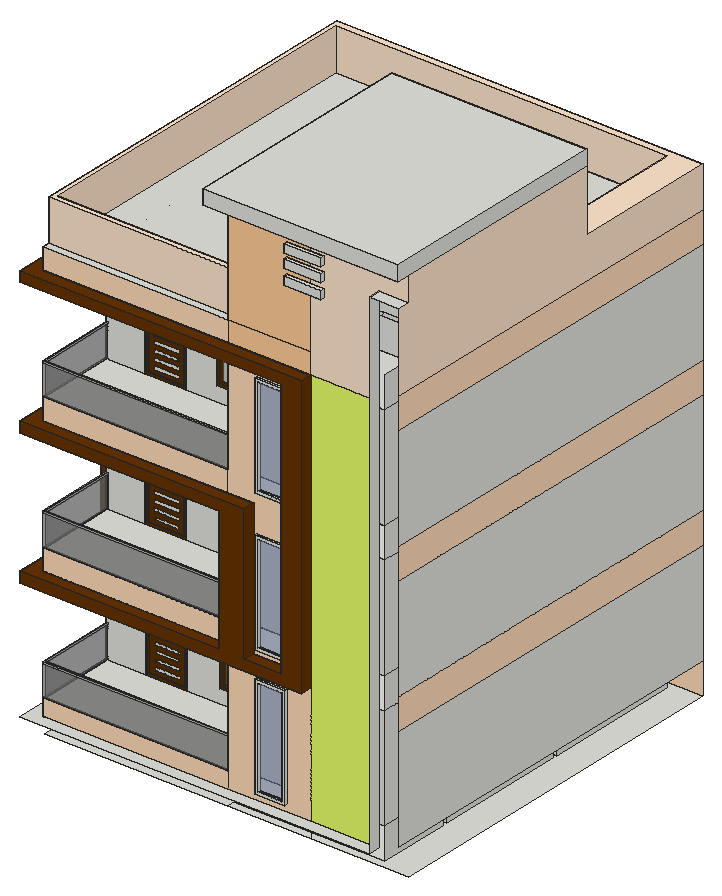
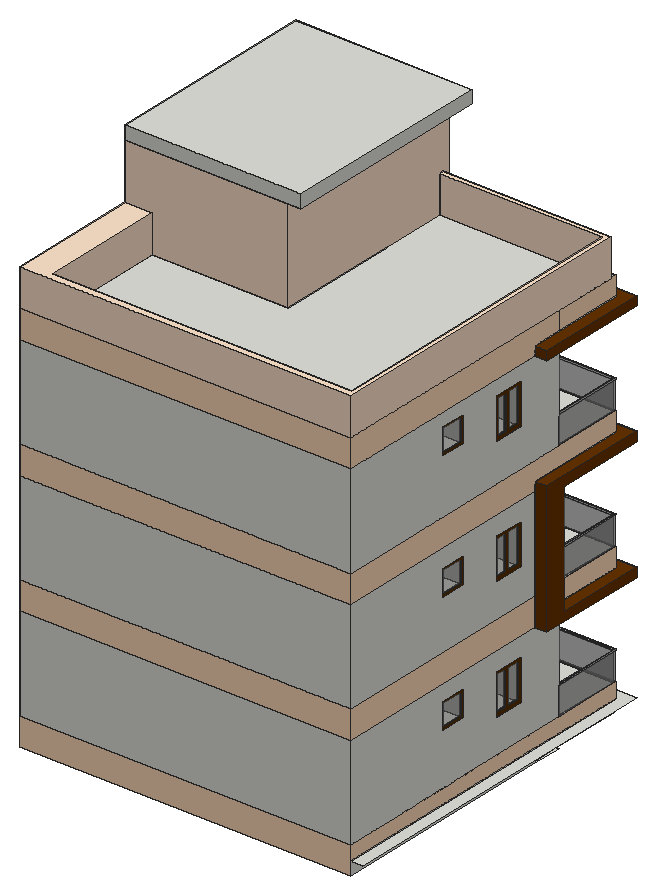
# SketchUp Ruby script. Lengths in inches.
U = 1.inch
M = Sketchup.active_model
def pt(a) = Geom::Point3d.new(a.map { |v| v * U })
def face(e, loops, mat)
  f = e.add_face(loops[0].map { |a| pt(a) })
  loops[1..].each { |l| e.add_face(l.map { |a| pt(a) }).erase! }
  f.material = f.back_material = mat if mat
  f
end
# faces: each face lists its corners as indices into pts; further lists are holes
def faces(e, pts, list, mat = nil) = list.each { |f| face(e, (f[0].is_a?(Array) ? f : [f]).map { |l| l.map { |i| pts[i] } }, mat) }
# xy, xz, yz: faces in a plane at the given z, y or x. An outline is a flat list of corners, or four numbers for a rectangle; further outlines are holes
def ring(l) = l.size == 4 ? [[l[0], l[1]], [l[2], l[1]], [l[2], l[3]], [l[0], l[3]]] : l.each_slice(2).to_a
def flat(e, list, mat, &to3) = list.each { |f| face(e, (f[0].is_a?(Array) ? f : [f]).map { |l| ring(l).map { |u, v| to3.(u, v) } }, mat) }
def xy(e, z, list, mat = nil) = flat(e, list, mat) { |x, y| [x, y, z] }
def xz(e, y, list, mat = nil) = flat(e, list, mat) { |x, z| [x, y, z] }
def yz(e, x, list, mat = nil) = flat(e, list, mat) { |y, z| [x, y, z] }
def lines(e, pts, list) = list.each { |a, b| e.add_line(pt(pts[a]), pt(pts[b])) }
# prism: a flat outline (further loops are holes) pulled along v
def prism(e, loops, v, mat = nil)
  f = face(e, loops, mat); d = Geom::Vector3d.new(v.map { |x| x * U })
  f.pushpull(f.normal.samedirection?(d) ? d.length : -d.length)
end
def box(e, o, s, mat = nil) = prism(e, [[o, [o[0] + s[0], o[1], o[2]], [o[0] + s[0], o[1] + s[1], o[2]], [o[0], o[1] + s[1], o[2]]]], [0, 0, s[2]], mat)
def at(x, y, z, deg = 0) = Geom::Transformation.translation(pt([x, y, z])) * Geom::Transformation.rotation(ORIGIN, Z_AXIS, deg.degrees)
def axes(o, x, y, z) = Geom::Transformation.new([*x, 0, *y, 0, *z, 0, *pt(o).to_a, 1])
def part(name) = M.definitions.add(name)
# library, detail: a bought-in or finely detailed component or shape, given as its bounding box
def library(name, o, s) = part(name).tap { |d| box(d.entities, o, s) }
def detail(e, o, s) = box(e.add_group.entities, o, s)
def put(e, d, t, mat = nil) = e.add_instance(d, t).tap { |i| i.material = mat if mat }
def group(e, t, mat = nil) = e.add_group.tap { |g| g.transformation = t; g.material = mat if mat }.entities
root = M.entities
M.materials.add("[0027_PeachPuff]").color = [255, 218, 185]
M.materials.add("[Aluminum]").color = [179, 179, 179]
M.materials.add("[Color A08]").color = [89, 48, 0]
M.materials.add("[Color C01]").color = [255, 229, 204]
M.materials.add("[Color C02]").color = [255, 204, 153]
M.materials.add("[Color C08]").color = [102, 51, 0]
M.materials.add("[Rectangles Running 4x1]").color = [231, 255, 106]
M.materials.add("[Translucent Glass Gray]").color = [128, 128, 128]
M.materials["[Translucent Glass Gray]"].alpha = 0.5
M.materials.add("[Translucent Glass Sky Reflection]").color = [126, 138, 183]
M.materials["[Translucent Glass Sky Reflection]"].alpha = 0.52
c1 = part("Group\#2")
xy(c1.entities,0,[[0,0,48,6.0625]],"[Color A08]")
xy(c1.entities,2.37,[[2.37,2.1875,45.63,6.0625]])
xy(c1.entities,2.37,[[2.37,0,45.63,2.1875]],"[Color A08]")
xy(c1.entities,81.63,[[2.37,2.1875,45.63,6.0625]])
xy(c1.entities,81.63,[[2.37,0,45.63,2.1875]],"[Color A08]")
xy(c1.entities,84,[[0,0,48,6.0625]],"[Color A08]")
xz(c1.entities,0,[[[0,0,48,84],[2.37,2.37,45.63,81.63]]],"[Color A08]")
xz(c1.entities,2.1875,[[9.64,6.54,37.83,9.91],[9.64,15.35,37.83,18.72],[9.64,24.16,37.83,27.54],[9.64,32.97,37.83,36.35],[9.64,41.79,37.83,45.16],
  [9.64,50.6,37.83,53.97],[9.64,59.41,37.83,62.79],[9.64,68.22,37.83,71.6]])
xz(c1.entities,2.1875,[[[2.37,2.37,45.63,81.63],[9.64,68.22,37.83,71.6],[9.64,59.41,37.83,62.79],[9.64,50.6,37.83,53.97],[9.64,41.79,37.83,45.16],[9.64,32.97,37.83,36.35],[9.64,24.16,37.83,27.54],[9.64,15.35,37.83,18.72],[9.64,6.54,37.83,9.91]]],"[Color A08]")
xz(c1.entities,6.0625,[[[0,0,48,84],[2.37,2.37,45.63,81.63]],[2.37,2.37,45.63,81.63]],"[Color A08]")
yz(c1.entities,0,[[0,0,6.0625,84]],"[Color A08]")
yz(c1.entities,2.37,[[2.1875,2.37,6.0625,81.63]])
yz(c1.entities,2.37,[[0,2.37,2.1875,81.63]],"[Color A08]")
yz(c1.entities,45.63,[[2.1875,2.37,6.0625,81.63]])
yz(c1.entities,45.63,[[0,2.37,2.1875,81.63]],"[Color A08]")
yz(c1.entities,48,[[0,0,6.0625,84]],"[Color A08]")
c2 = part("Group\#1")
xy(c2.entities,0,[[0,0,54.25,4.125]],"[Color A08]")
xy(c2.entities,2.45,[[2.45,0,51.8,4.125]],"[Color A08]")
xy(c2.entities,43.87,[[2.45,0,51.8,4.125]],"[Color A08]")
xy(c2.entities,46.3125,[[0,0,54.25,4.125]],"[Color A08]")
xz(c2.entities,0,[[[0,0,54.25,46.3125],[2.45,2.45,51.8,43.87]]],"[Color A08]")
xz(c2.entities,4.125,[[[0,0,54.25,46.3125],[2.45,2.45,51.8,43.87]]],"[Color A08]")
xz(c2.entities,4.125,[[2.45,2.45,51.8,43.87]],"[Translucent Glass Gray]")
yz(c2.entities,0,[[0,0,4.125,46.3125]],"[Color A08]")
yz(c2.entities,2.45,[[0,2.45,4.125,43.87]],"[Color A08]")
yz(c2.entities,51.8,[[0,2.45,4.125,43.87]],"[Color A08]")
yz(c2.entities,54.25,[[0,0,4.125,46.3125]],"[Color A08]")
c3 = part("Group\#3")
xy(c3.entities,0,[[0,0,1.5,39.25],[1.5,0,2.8125,39.25]],"[Color A08]")
xy(c3.entities,3.22,[[0,3.22,1.5,19.0625],[1.5,3.22,2.8125,19.0625],[1.5,19.0625,2.8125,22.29],[0,22.29,1.5,36.03],[1.5,22.29,2.8125,36.03]],"[Color A08]")
xy(c3.entities,36.03,[[0,3.22,1.5,19.0625],[1.5,3.22,2.8125,19.0625],[0,19.0625,1.5,22.29],[1.5,19.0625,2.8125,22.29],[0,22.29,1.5,36.03],
  [1.5,22.29,2.8125,36.03]],"[Color A08]")
xy(c3.entities,39.25,[[0,0,1.5,39.25],[1.5,0,2.8125,39.25]],"[Color A08]")
xz(c3.entities,0,[[0,0,1.5,39.25],[1.5,0,2.8125,39.25]],"[Color A08]")
xz(c3.entities,3.22,[[0,3.22,1.5,36.03],[1.5,3.22,2.8125,36.03]],"[Color A08]")
xz(c3.entities,19.0625,[[0,3.22,1.5,36.03],[1.5,3.22,2.8125,36.03]],"[Color A08]")
xz(c3.entities,22.29,[[0,3.22,1.5,36.03],[1.5,3.22,2.8125,36.03]],"[Color A08]")
xz(c3.entities,36.03,[[0,3.22,1.5,36.03],[1.5,3.22,2.8125,36.03]],"[Color A08]")
xz(c3.entities,39.25,[[0,0,1.5,39.25],[1.5,0,2.8125,39.25]],"[Color A08]")
yz(c3.entities,0,[[[0,0,39.25,39.25],[3.22,3.22,19.0625,36.03],[22.29,3.22,36.03,36.03]]],"[Color A08]")
yz(c3.entities,1.5,[[[0,0,39.25,39.25],[3.22,3.22,36.03,36.03]],[19.0625,3.22,22.29,36.03]],"[Color A08]")
yz(c3.entities,1.5,[[3.22,3.22,19.0625,36.03],[22.29,3.22,36.03,36.03]],"[Translucent Glass Gray]")
yz(c3.entities,2.8125,[[[0,0,39.25,39.25],[3.22,3.22,36.03,36.03]],[19.0625,3.22,22.29,36.03]],"[Color A08]")
c4 = part("Group\#4")
xy(c4.entities,0,[[0,0,1.5,39.25],[1.5,0,2.8125,39.25]],"[Color A08]")
xy(c4.entities,3.22,[[0,3.22,1.5,36.03],[1.5,3.22,2.8125,36.03]],"[Color A08]")
xy(c4.entities,36.03,[[0,3.22,1.5,36.03],[1.5,3.22,2.8125,36.03]],"[Color A08]")
xy(c4.entities,39.25,[[0,0,1.5,39.25],[1.5,0,2.8125,39.25]],"[Color A08]")
xz(c4.entities,0,[[0,0,1.5,39.25],[1.5,0,2.8125,39.25]],"[Color A08]")
xz(c4.entities,3.22,[[0,3.22,1.5,36.03],[1.5,3.22,2.8125,36.03]],"[Color A08]")
xz(c4.entities,36.03,[[0,3.22,1.5,36.03],[1.5,3.22,2.8125,36.03]],"[Color A08]")
xz(c4.entities,39.25,[[0,0,1.5,39.25],[1.5,0,2.8125,39.25]],"[Color A08]")
yz(c4.entities,0,[[[0,0,39.25,39.25],[3.22,3.22,36.03,36.03]]],"[Color A08]")
yz(c4.entities,1.5,[[[0,0,39.25,39.25],[3.22,3.22,36.03,36.03]]],"[Color A08]")
yz(c4.entities,1.5,[[3.22,3.22,36.03,36.03]],"[Translucent Glass Gray]")
yz(c4.entities,2.8125,[[[0,0,39.25,39.25],[3.22,3.22,36.03,36.03]]],"[Color A08]")
xy(root,594,[[[239.3125,57,239.3125,66,414,66,414,149.375,27.5,149.375,27.5,187.1,24.5,187.1,24.5,483,448.4375,483,448.4375,57],[66,155.375,239.3125,155.375,239.3125,314.6875,414,314.6875,414,474,66,474],[245.3125,155.375,414,308.6875]],[27.5,57,27.5,149.375,414,149.375,414,66,239.3125,66,239.3125,57],[24.5,149.375,27.5,187.1]])
xy(root,606,[[24.5,57,27.5,187.1]])
xy(root,611.375,[[9.1875,43.625,414.23,43.625,414.23,57,24.5,57,24.5,483,9.1875,483]])
xy(root,619.3,[[273.13,54,307.66,57]])
xy(root,622.35,[[276.18,54,304.61,57]])
xy(root,624,[[66,155.375,66,474,414,474,414,314.6875,239.3125,314.6875,239.3125,155.375]])
xy(root,630,[[24.5,57,24.5,149.375,26.5,149.375,26.5,59,239.3125,59,239.3125,57],[26.5,59,239.3125,59,239.3125,66,414,66,414,149.375,118.3,149.375,118.3,155.375,70.3,155.375,70.3,149.375,26.5,149.375],[66,155.375,239.3125,155.375,239.3125,314.6875,414,314.6875,414,474,66,474],[245.3125,155.375,414,308.6875]])
xy(root,645.46,[[156.65,149.375,230.4,155.375]])
xy(root,666,[[24.5,57,24.5,149.375,26.5,149.375,26.5,59,239.3125,59,239.3125,57]],"[Aluminum]")
xy(root,668,[[24.5,57,239.3125,57,239.3125,59,26.5,59,26.5,149.375,24.5,149.375]],"[Aluminum]")
xy(root,672.38,[[24.5,208.14,66,249.33]])
xy(root,696.05,[[24.5,301.46,66,335.96]])
xy(root,713.65,[[156.65,149.375,230.4,155.375]])
xy(root,714,[[70.3,149.375,118.3,155.375]])
xy(root,726.26,[[24.5,208.14,66,249.33]])
xy(root,730.55,[[24.5,301.46,66,335.96]])
xy(root,735.41,[[276.18,54,277.97,57],[277.97,54,280.16,57],[280.16,54,304.61,57]])
xy(root,738.46,[[273.13,54,307.66,57]])
xy(root,750,[[24.5,57,24.5,149.375,414,149.375,414,66,239.3125,66,239.3125,57]])
xy(root,750,[[9.1875,43.625,9.1875,187.1,24.5,187.1,24.5,57,335.42,57,335.42,43.625]],"[Color C08]")
xy(root,762,[[9.1875,43.625,239.3125,43.625,239.3125,57,24.5,57,24.5,160.8,9.1875,160.8],[268.87,43.625,310.94,57]],"[Color C08]")
xy(root,768.49,[[273.13,54,307.66,57]])
xy(root,771.53,[[276.18,54,304.61,57]])
xy(root,780,[[245.3125,155.375,414,308.6875]])
xy(root,780.875,[[66,155.375,66,474,414,474,414,314.6875,239.3125,314.6875,239.3125,155.375]])
xy(root,786,[[24.5,57,24.5,149.375,26.5,149.375,26.5,59,239.3125,59,239.3125,57],[26.5,59,239.3125,59,239.3125,66,414,66,414,149.375,117.05,149.375,117.05,155.375,69.05,155.375,69.05,149.375,26.5,149.375],[66,155.375,239.3125,155.375,239.3125,314.6875,414,314.6875,414,474,66,474],[245.3125,155.375,414,308.6875]])
xy(root,799.96,[[155.08,149.375,228.83,155.375]])
xy(root,822,[[24.5,57,24.5,149.375,26.5,149.375,26.5,59,239.3125,59,239.3125,57]],"[Aluminum]")
xy(root,824,[[24.5,57,239.3125,57,239.3125,59,26.5,59,26.5,149.375,24.5,149.375]],"[Aluminum]")
xy(root,828.51,[[24.5,208.14,66,249.33]])
xy(root,848.8,[[24.5,301.46,66,335.96]])
xy(root,868.15,[[155.08,149.375,228.83,155.375]])
xy(root,870,[[69.05,149.375,117.05,155.375]])
xy(root,882.38,[[24.5,208.14,66,249.33]])
xy(root,883.3,[[24.5,301.46,66,335.96]])
xy(root,884.6,[[276.18,54,304.61,57]])
xy(root,887.64,[[273.13,54,307.66,57]])
xy(root,906,[[24.5,57,24.5,149.375,414,149.375,414,66,239.3125,66,239.3125,57]])
xy(root,906,[[9.1875,43.625,9.1875,160.8,24.5,160.8,24.5,57,239.3125,57,239.3125,43.625]],"[Color C08]")
xy(root,918,[[9.1875,43.625,268.87,43.625,268.87,57,24.5,57,24.5,187.1,9.1875,187.1]],"[Color C08]")
xy(root,931.68,[[273.13,54,307.66,57]])
xy(root,934.72,[[276.18,54,304.61,57]])
xy(root,938.8125,[[245.3125,155.375,414,308.6875]])
xy(root,940.125,[[66,155.375,66,474,414,474,414,314.6875,239.3125,314.6875,239.3125,155.375]])
xy(root,942,[[24.5,57,24.5,149.375,26.5,149.375,26.5,59,239.3125,59,239.3125,57],[26.5,59,239.3125,59,239.3125,149.375,117.3,149.375,117.3,155.375,69.3,155.375,69.3,149.375,26.5,149.375],[239.3125,66,414,149.375],[66,155.375,239.3125,155.375,239.3125,314.6875,414,314.6875,414,474,66,474],[245.3125,155.375,414,308.6875]])
xy(root,958.16,[[152.67,149.375,226.42,155.375]])
xy(root,978,[[24.5,57,24.5,149.375,26.5,149.375,26.5,59,239.3125,59,239.3125,57]],"[Aluminum]")
xy(root,980,[[24.5,57,239.3125,57,239.3125,59,26.5,59,26.5,149.375,24.5,149.375]],"[Aluminum]")
xy(root,990.07,[[24.5,208.14,66,249.33]])
xy(root,1011.55,[[24.5,301.46,66,335.96]])
xy(root,1026,[[69.3,149.375,117.3,155.375]])
xy(root,1026.34,[[152.67,149.375,226.42,155.375]])
xy(root,1043.95,[[24.5,208.14,66,249.33]])
xy(root,1046.05,[[24.5,301.46,66,335.96]])
xy(root,1047.78,[[276.18,54,281.61,57],[281.61,54,304.61,57]])
xy(root,1050.83,[[273.13,54,307.66,57]])
xy(root,1062,[[24.5,57,24.5,149.375,414,149.375,414,66,239.3125,66,239.3125,57]])
xy(root,1062,[[9.1875,43.625,9.1875,187.1,24.5,187.1,24.5,57,310.94,57,310.94,43.625]],"[Color C08]")
xy(root,1074,[[9.1875,43.625,335.42,43.625,335.42,57,24.5,57,24.5,187.1,9.1875,187.1]],"[Color C08]")
xy(root,1092,[[66,155.375,66,474,414,474,414,314.6875,239.3125,314.6875,239.3125,155.375]])
xy(root,1092.125,[[245.3125,155.375,414,308.6875]])
xy(root,1098,[[24.5,57,239.3125,66],[24.5,66,24.5,483,240,483,240,474,30.5,474,30.5,72,239.3125,72,239.3125,66],[30.5,72,239.3125,72,239.3125,314.6875,414,314.6875,414,474,30.5,474],[245.3125,155.375,414,308.6875]])
xy(root,1146,[[24.5,66,239.3125,66,239.3125,72,30.5,72,30.5,474,414,474,414,314.6875,448.4375,314.6875,448.4375,483,24.5,483]],"[Color C01]")
xy(root,1160.22,[[307.94,52.3125,350.75,57]])
xy(root,1169.53,[[307.94,52.3125,350.75,57]])
xy(root,1177.59,[[307.94,52.3125,350.75,57]])
xy(root,1186.9,[[307.94,52.3125,350.75,57]])
xy(root,1188.8,[[414.23,43.625,448.4375,57]])
xy(root,1193.59,[[307.94,52.3125,350.75,57]])
xy(root,1202.9,[[307.94,52.3125,350.75,57]])
xy(root,1212,[[245.3125,155.375,414,308.6875]])
xy(root,1218,[[222.625,41.1875,222.625,314.6875,239.3125,314.6875,239.3125,57,448.4375,57,448.4375,41.1875],[239.3125,57,448.4375,314.6875]])
xy(root,1235,[[222.625,41.1875,448.4375,314.6875]])
xz(root,41.1875,[[222.625,1218,448.4375,1235]])
xz(root,43.625,[[9.1875,750,335.42,750,335.42,1074,9.1875,1074,9.1875,1062,310.94,1062,310.94,762,268.87,762,268.87,918,9.1875,918,9.1875,906,239.3125,906,239.3125,762,9.1875,762]],"[Color C08]")
xz(root,52.3125,[[307.94,1160.22,350.75,1169.53],[307.94,1177.59,350.75,1186.9],[307.94,1193.59,350.75,1202.9]])
xz(root,54,[[[273.13,619.3,307.66,738.46],[276.18,622.35,304.61,735.41]],[[273.13,768.49,307.66,887.64],[276.18,771.53,304.61,884.6]],[[273.13,931.68,307.66,1050.83],[276.18,934.72,304.61,1047.78]]])
xz(root,57,[[24.5,606,27.5,611.375],[[273.13,619.3,307.66,738.46],[276.18,622.35,304.61,735.41]],[24.5,750,24.5,762,239.3125,762,239.3125,906,24.5,906,24.5,918,268.87,918,268.87,762,310.94,762,310.94,1062,24.5,1062,24.5,1074,335.42,1074,335.42,750],[[273.13,768.49,307.66,887.64],[276.18,771.53,304.61,884.6]],[[273.13,931.68,307.66,1050.83],[276.18,934.72,304.61,1047.78]],
  [307.94,1160.22,350.75,1169.53],[307.94,1177.59,350.75,1186.9],[307.94,1193.59,350.75,1202.9]])
xz(root,57,[[24.5,611.375,239.3125,630],[[239.3125,611.375,335.42,750],[273.13,619.3,307.66,738.46]],[24.5,762,239.3125,786],[[268.87,762,310.94,762,310.94,1062,239.3125,1062,239.3125,918,268.87,918],[273.13,768.49,307.66,887.64],[273.13,931.68,307.66,1050.83]],[24.5,918,239.3125,942],
  [24.5,1074,239.3125,1098]],"[0027_PeachPuff]")
xz(root,57,[[24.5,666,239.3125,668],[24.5,822,239.3125,824],[24.5,978,239.3125,980]],"[Aluminum]")
xz(root,57,[[335.42,1074,414.23,1074,414.23,1188.8,448.4375,1188.8,448.4375,1218,335.42,1218,335.42,1202.9,350.75,1202.9,350.75,1193.59,335.42,1193.59,335.42,1186.9,350.75,1186.9,350.75,1177.59,335.42,1177.59,335.42,1169.53,350.75,1169.53,350.75,1160.22,335.42,1160.22]],"[Color C01]")
xz(root,57,[[239.3125,1074,335.42,1098],[239.3125,1098,335.42,1098,335.42,1160.22,307.94,1160.22,307.94,1169.53,335.42,1169.53,335.42,1177.59,307.94,1177.59,307.94,1186.9,335.42,1186.9,335.42,1193.59,307.94,1193.59,307.94,1202.9,335.42,1202.9,335.42,1218,239.3125,1218]],"[Color C02]")
xz(root,57,[[335.42,611.375,414.23,1074]],"[Rectangles Running 4x1]")
xz(root,57,[[24.5,630,239.3125,666],[24.5,786,239.3125,822],[24.5,942,239.3125,978]],"[Translucent Glass Gray]")
xz(root,57,[[276.18,622.35,304.61,735.41],[276.18,771.53,304.61,884.6],[276.18,934.72,304.61,1047.78]],"[Translucent Glass Sky Reflection]")
xz(root,59,[[26.5,666,239.3125,668],[26.5,822,239.3125,824],[26.5,978,239.3125,980]],"[Aluminum]")
xz(root,59,[[26.5,630,239.3125,666],[26.5,786,239.3125,822],[26.5,942,239.3125,978]],"[Translucent Glass Gray]")
xz(root,66,[[239.3125,630,414,750],[239.3125,786,414,906],[239.3125,942,414,1062]])
xz(root,66,[[24.5,1098,239.3125,1146]],"[Color C01]")
xz(root,72,[[30.5,1098,239.3125,1146]],"[Color C01]")
xz(root,149.375,[[239.3125,594,414,630],[24.5,630,26.5,666],[[26.5,630,70.3,630,70.3,714,118.3,714,118.3,630,414,630,414,750,24.5,750,24.5,668,26.5,668],[156.65,645.46,230.4,713.65]],[239.3125,750,414,786],[24.5,786,26.5,822],
  [[26.5,786,69.05,786,69.05,870,117.05,870,117.05,786,414,786,414,906,24.5,906,24.5,824,26.5,824],[155.08,799.96,228.83,868.15]],[239.3125,906,414,942],[24.5,942,26.5,978],[[26.5,942,69.3,942,69.3,1026,117.3,1026,117.3,942,414,942,414,1062,24.5,1062,24.5,980,26.5,980],[152.67,958.16,226.42,1026.34]],[239.3125,1062,414,1098]])
xz(root,149.375,[[24.5,666,26.5,668],[24.5,822,26.5,824],[24.5,978,26.5,980]],"[Aluminum]")
xz(root,155.375,[[66,594,239.3125,624],[245.3125,594,298.66,630],[298.66,594,307.22,630],[307.22,594,414,630],[66,624,70.3,630],
  [70.3,624,118.3,630],[118.3,624,233.875,630],[233.875,624,239.3125,630],[[66,630,66,750,239.3125,750,239.3125,630,118.3,630,118.3,714,70.3,714,70.3,630],[156.65,645.46,230.4,713.65]],[245.3125,630,414,750],
  [66,750,239.3125,780.875],[245.3125,750,414,780],[245.3125,780,320.47,786],[320.47,780,329.66,786],[329.66,780,414,786],
  [66,780.875,69.05,786],[69.05,780.875,117.05,786],[117.05,780.875,233.3125,786],[233.3125,780.875,239.3125,786],[[66,786,66,906,239.3125,906,239.3125,786,117.05,786,117.05,870,69.05,870,69.05,786],[155.08,799.96,228.83,868.15]],
  [245.3125,786,414,906],[66,906,239.3125,940.125],[245.3125,906,414,938.8125],[245.3125,938.8125,363.6,942],[363.6,938.8125,371.03,942],
  [371.03,938.8125,414,942],[66,940.125,69.3,942],[69.3,940.125,117.3,942],[117.3,940.125,232.0625,942],[232.0625,940.125,239.3125,942],
  [[66,942,66,1062,239.3125,1062,239.3125,942,117.3,942,117.3,1026,69.3,1026,69.3,942],[152.67,958.16,226.42,1026.34]],[245.3125,942,414,1062],[66,1062,239.3125,1092],[245.3125,1062,414,1092.125],[245.3125,1092.125,329.66,1098],
  [329.66,1092.125,340.1875,1098],[340.1875,1092.125,414,1098],[245.3125,1098,414,1212]])
xz(root,160.8,[[9.1875,762,24.5,906]],"[Color C08]")
xz(root,187.1,[[24.5,594,27.5,606]])
xz(root,187.1,[[9.1875,750,24.5,918],[9.1875,1062,24.5,1074]],"[Color C08]")
xz(root,208.14,[[24.5,672.38,66,726.26],[24.5,828.51,66,882.38],[24.5,990.07,66,1043.95]])
xz(root,249.33,[[24.5,672.38,66,726.26],[24.5,828.51,66,882.38],[24.5,990.07,66,1043.95]])
xz(root,301.46,[[24.5,696.05,66,730.55],[24.5,848.8,66,883.3],[24.5,1011.55,66,1046.05]])
xz(root,308.6875,[[245.3125,594,414,630],[245.3125,630,414,750],[245.3125,750,414,780],[245.3125,780,414,786],[245.3125,786,414,906],
  [245.3125,906,414,938.8125],[245.3125,938.8125,414,942],[245.3125,942,414,1062],[245.3125,1062,414,1092.125],[245.3125,1092.125,414,1098],
  [245.3125,1098,414,1212]])
xz(root,314.6875,[[239.3125,594,414,624],[239.3125,624,414,630],[239.3125,630,414,750],[239.3125,750,414,780.875],[239.3125,780.875,414,786],
  [239.3125,786,414,906],[239.3125,906,414,940.125],[239.3125,940.125,414,942],[239.3125,942,414,1062],[239.3125,1062,414,1092],
  [239.3125,1092,414,1098],[222.625,1218,448.4375,1235]])
xz(root,314.6875,[[239.3125,1098,239.3125,1218,448.4375,1218,448.4375,1146,414,1146,414,1098]],"[Color C01]")
xz(root,335.96,[[24.5,696.05,66,730.55],[24.5,848.8,66,883.3],[24.5,1011.55,66,1046.05]])
xz(root,474,[[66,594,414,624],[66,624,414,630],[66,630,414,750],[66,750,414,780.875],[66,780.875,414,786],
  [66,786,414,906],[66,906,414,940.125],[66,940.125,414,942],[66,942,414,1062],[66,1062,414,1092],
  [66,1092,240,1098],[240,1092,414,1098]])
xz(root,474,[[30.5,1098,414,1146]],"[Color C01]")
xz(root,483,[[24.5,630,448.4375,750],[24.5,786,448.4375,906],[24.5,942,448.4375,1062]])
xz(root,483,[[24.5,594,448.4375,630],[24.5,750,448.4375,786],[24.5,906,448.4375,942],[24.5,1062,448.4375,1098]],"[0027_PeachPuff]")
xz(root,483,[[24.5,1098,448.4375,1146]],"[Color C01]")
yz(root,9.1875,[[43.625,750,43.625,762,160.8,762,160.8,906,43.625,906,43.625,918,187.1,918,187.1,750],[43.625,1062,187.1,1074]],"[Color C08]")
yz(root,24.5,[[187.1,594,483,611.375],[57,606,187.1,611.375],[[149.375,630,483,750],[208.14,672.38,249.33,726.26],[301.46,696.05,335.96,730.55]],[57,750,187.1,750,187.1,918,57,918,57,906,160.8,906,160.8,762,57,762],[[187.1,786,483,906],[208.14,828.51,249.33,882.38],[301.46,848.8,335.96,883.3]],
  [[149.375,942,483,1062],[208.14,990.07,249.33,1043.95],[301.46,1011.55,335.96,1046.05]],[57,1062,187.1,1074]])
yz(root,24.5,[[57,611.375,483,630],[187.1,750,483,786],[57,762,57,786,149.375,786,149.375,906,160.8,906,160.8,762],[187.1,906,187.1,918,57,918,57,942,483,942,483,906],[187.1,1062,187.1,1074,149.375,1074,149.375,1098,483,1098,483,1062],
  [57,1074,149.375,1098]],"[0027_PeachPuff]")
yz(root,24.5,[[57,666,149.375,668],[57,822,149.375,824],[57,978,149.375,980]],"[Aluminum]")
yz(root,24.5,[[66,1098,483,1146]],"[Color C01]")
yz(root,24.5,[[57,630,149.375,666],[57,786,149.375,822],[57,942,149.375,978]],"[Translucent Glass Gray]")
yz(root,26.5,[[59,666,149.375,668],[59,822,149.375,824],[59,978,149.375,980]],"[Aluminum]")
yz(root,26.5,[[59,630,149.375,666],[59,786,149.375,822],[59,942,149.375,978]],"[Translucent Glass Gray]")
yz(root,30.5,[[72,1098,474,1146]],"[Color C01]")
yz(root,66,[[155.375,594,474,624],[155.375,624,474,630],[[155.375,630,474,750],[208.14,672.38,249.33,726.26],[301.46,696.05,335.96,730.55]],[155.375,750,474,780.875],[155.375,780.875,474,786],
  [[155.375,786,474,906],[208.14,828.51,249.33,882.38],[301.46,848.8,335.96,883.3]],[155.375,906,474,940.125],[155.375,940.125,474,942],[[155.375,942,474,1062],[208.14,990.07,249.33,1043.95],[301.46,1011.55,335.96,1046.05]],[155.375,1062,474,1092]])
yz(root,69.05,[[149.375,786,155.375,870]])
yz(root,69.3,[[149.375,942,155.375,1026]])
yz(root,70.3,[[149.375,630,155.375,714]])
yz(root,117.05,[[149.375,786,155.375,870]])
yz(root,117.3,[[149.375,942,155.375,1026]])
yz(root,118.3,[[149.375,630,155.375,714]])
yz(root,152.67,[[149.375,958.16,155.375,1026.34]])
yz(root,155.08,[[149.375,799.96,155.375,868.15]])
yz(root,156.65,[[149.375,645.46,155.375,713.65]])
yz(root,222.625,[[41.1875,1218,314.6875,1235]])
yz(root,226.42,[[149.375,958.16,155.375,1026.34]])
yz(root,228.83,[[149.375,799.96,155.375,868.15]])
yz(root,230.4,[[149.375,645.46,155.375,713.65]])
yz(root,239.3125,[[155.375,594,314.6875,624],[155.375,624,314.6875,630],[57,630,59,666],[59,630,59,668,57,668,57,750,66,750,66,630],[155.375,630,314.6875,750],
  [155.375,750,314.6875,780.875],[155.375,780.875,314.6875,786],[57,786,59,822],[59,786,59,824,57,824,57,906,66,906,66,786],[155.375,786,314.6875,906],
  [155.375,906,314.6875,940.125],[155.375,940.125,314.6875,942],[57,942,59,978],[59,942,59,980,57,980,57,1062,66,1062,66,942],[155.375,942,314.6875,1062],
  [155.375,1062,314.6875,1092],[155.375,1092,314.6875,1098],[66,1098,72,1146]])
yz(root,239.3125,[[57,666,59,668],[57,822,59,824],[57,978,59,980]],"[Aluminum]")
yz(root,239.3125,[[57,1098,57,1218,314.6875,1218,314.6875,1098,72,1098,72,1146,66,1146,66,1098]],"[Color C01]")
yz(root,239.3125,[[43.625,762,57,906]],"[Color C08]")
yz(root,245.3125,[[155.375,594,308.6875,630],[155.375,630,308.6875,750],[155.375,750,308.6875,780],[155.375,780,308.6875,786],[155.375,786,308.6875,906],
  [155.375,906,308.6875,938.8125],[155.375,938.8125,308.6875,942],[155.375,942,308.6875,1062],[155.375,1062,308.6875,1092.125],[155.375,1092.125,308.6875,1098],
  [155.375,1098,308.6875,1212]])
yz(root,268.87,[[43.625,762,57,918]],"[Color C08]")
yz(root,273.13,[[54,619.3,57,738.46],[54,768.49,57,887.64],[54,931.68,57,1050.83]])
yz(root,276.18,[[54,622.35,57,735.41],[54,771.53,57,884.6],[54,934.72,57,1047.78]])
yz(root,304.61,[[54,622.35,57,735.41],[54,771.53,57,884.6],[54,934.72,57,1047.78]])
yz(root,307.66,[[54,619.3,57,738.46],[54,768.49,57,887.64],[54,931.68,57,1050.83]])
yz(root,307.94,[[52.3125,1160.22,57,1169.53],[52.3125,1177.59,57,1186.9],[52.3125,1193.59,57,1202.9]])
yz(root,310.94,[[43.625,762,57,1062]],"[Color C08]")
yz(root,335.42,[[43.625,750,57,1074]],"[Color C08]")
yz(root,350.75,[[52.3125,1160.22,57,1169.53],[52.3125,1177.59,57,1186.9],[52.3125,1193.59,57,1202.9]])
yz(root,414,[[66,594,149.375,630],[155.375,594,308.6875,630],[314.6875,594,474,624],[314.6875,624,474,630],[66,630,149.375,750],
  [155.375,630,308.6875,750],[314.6875,630,474,750],[66,750,149.375,786],[155.375,750,308.6875,780],[314.6875,750,474,780.875],
  [155.375,780,308.6875,786],[314.6875,780.875,474,786],[66,786,149.375,906],[155.375,786,308.6875,906],[314.6875,786,474,906],
  [66,906,149.375,942],[155.375,906,308.6875,938.8125],[314.6875,906,474,940.125],[155.375,938.8125,308.6875,942],[314.6875,940.125,474,942],
  [66,942,149.375,1062],[155.375,942,308.6875,1062],[314.6875,942,474,1062],[66,1062,149.375,1098],[155.375,1062,308.6875,1092.125],
  [314.6875,1062,474,1092],[314.6875,1092,474,1098],[155.375,1092.125,308.6875,1098],[155.375,1098,308.6875,1212]])
yz(root,414,[[314.6875,1098,474,1146]],"[Color C01]")
yz(root,414.23,[[43.625,611.375,57,1188.8]])
yz(root,448.4375,[[43.625,630,483,750],[43.625,786,483,906],[43.625,942,483,1062],[41.1875,1218,314.6875,1235]])
yz(root,448.4375,[[43.625,750,483,786],[43.625,906,483,942],[43.625,1062,483,1098]],"[0027_PeachPuff]")
yz(root,448.4375,[[43.625,1098,483,1098,483,1146,314.6875,1146,314.6875,1218,57,1218,57,1188.8,43.625,1188.8]],"[Color C01]")
p = [[239.3125,66,594],[239.3125,66,630],[239.3125,66,750],[239.3125,66,786],[239.3125,66,906],[239.3125,66,942],
  [239.3125,66,1062],[239.3125,66,1098],[335.42,57,611.375],[335.42,57,594],[404.6875,155.375,1218],[404.6875,155.375,1212],
  [414,155.375,1212],[414,155.375,1218],[414,308.6875,1212],[414,308.6875,1218],[245.3125,155.375,1212],[245.3125,155.375,1218],
  [245.3125,308.6875,1212],[245.3125,308.6875,1218],[66,189.55,1098],[66,189.55,1092],[66,155.375,1092],[66,155.375,1098]]
lines(root,p,[[0,1],[2,3],[4,5],[6,7],[8,9],[10,11],[12,13],[14,15],[16,17],[18,19],[20,21],[22,23]])
put(root,c1,at(70.3,149.375,630))
put(root,c2,axes([156.65,149.375,645.46],[1.35945,0,0],[0,1,0],[0,0,1.47233]))
put(root,c3,axes([26.1875,208.14,672.38],[1,0,0],[0,1.04,0],[0,0,1.3635]))
put(root,c4,axes([25.12,301.46,696.05],[0.78,0,0],[0,0.897,0],[0,0,0.88312]))
put(root,c1,at(69.3,149.375,786))
put(root,c2,axes([155.08,149.375,799.96],[1.35945,0,0],[0,1,0],[0,0,1.47233]))
put(root,c3,axes([26.1875,208.14,828.51],[1,0,0],[0,1.04,0],[0,0,1.3635]))
put(root,c4,axes([25.12,301.46,848.8],[0.78,0,0],[0,0.897,0],[0,0,0.88312]))
put(root,c1,at(69.3,149.375,942))
put(root,c2,axes([152.67,149.375,958.16],[1.35945,0,0],[0,1,0],[0,0,1.47233]))
put(root,c3,axes([25.875,208.14,990.07],[1,0,0],[0,1.04,0],[0,0,1.3635]))
g1 = group(root,at(25.12,301.46,1011.55))
xy(g1,0,[[0,0,1.17,35.21],[1.17,0,2.19,35.21]],"[Color A08]")
xy(g1,2.84,[[0,2.89,1.17,32.32],[1.17,2.89,2.19,32.32]],"[Color A08]")
xy(g1,31.82,[[0,2.89,1.17,32.32],[1.17,2.89,2.19,32.32]],"[Color A08]")
xy(g1,34.66,[[0,0,1.17,35.21],[1.17,0,2.19,35.21]],"[Color A08]")
xz(g1,0,[[0,0,1.17,34.66],[1.17,0,2.19,34.66]],"[Color A08]")
xz(g1,2.89,[[0,2.84,1.17,31.82],[1.17,2.84,2.19,31.82]],"[Color A08]")
xz(g1,32.32,[[0,2.84,1.17,31.82],[1.17,2.84,2.19,31.82]],"[Color A08]")
xz(g1,35.21,[[0,0,1.17,34.66],[1.17,0,2.19,34.66]],"[Color A08]")
yz(g1,0,[[[0,0,35.21,34.66],[2.89,2.84,32.32,31.82]]],"[Color A08]")
yz(g1,1.17,[[[0,0,35.21,34.66],[2.89,2.84,32.32,31.82]]],"[Color A08]")
yz(g1,1.17,[[2.89,2.84,32.32,31.82]],"[Translucent Glass Gray]")
yz(g1,2.19,[[[0,0,35.21,34.66],[2.89,2.84,32.32,31.82]]],"[Color A08]")
